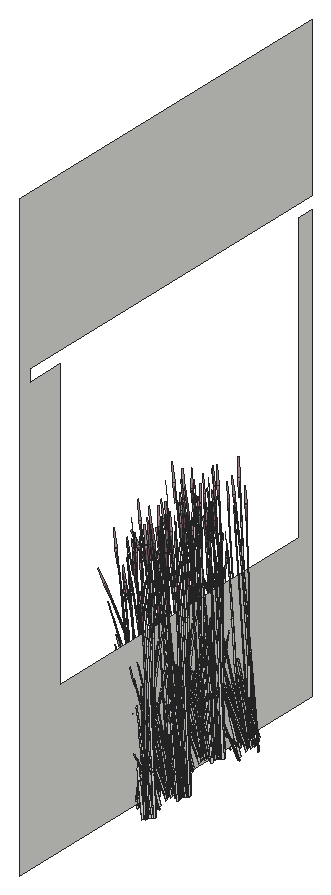
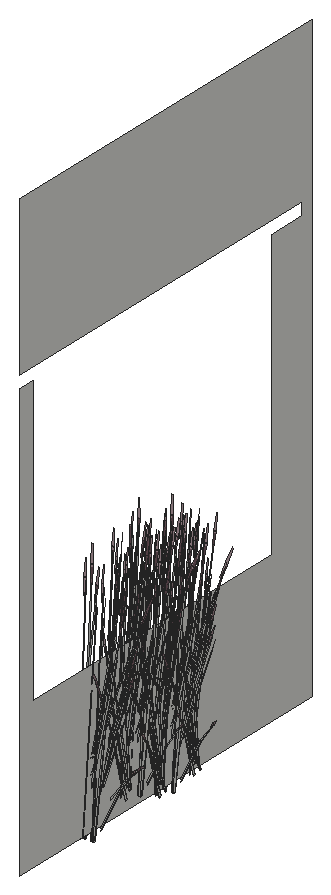
# SketchUp Ruby script. Lengths in inches.
U = 1.inch
M = Sketchup.active_model
def pt(a) = Geom::Point3d.new(a.map { |v| v * U })
def face(e, loops, mat)
  f = e.add_face(loops[0].map { |a| pt(a) })
  loops[1..].each { |l| e.add_face(l.map { |a| pt(a) }).erase! }
  f.material = f.back_material = mat if mat
  f
end
# faces: each face lists its corners as indices into pts; further lists are holes
def faces(e, pts, list, mat = nil) = list.each { |f| face(e, (f[0].is_a?(Array) ? f : [f]).map { |l| l.map { |i| pts[i] } }, mat) }
# xy, xz, yz: faces in a plane at the given z, y or x. An outline is a flat list of corners, or four numbers for a rectangle; further outlines are holes
def ring(l) = l.size == 4 ? [[l[0], l[1]], [l[2], l[1]], [l[2], l[3]], [l[0], l[3]]] : l.each_slice(2).to_a
def flat(e, list, mat, &to3) = list.each { |f| face(e, (f[0].is_a?(Array) ? f : [f]).map { |l| ring(l).map { |u, v| to3.(u, v) } }, mat) }
def xy(e, z, list, mat = nil) = flat(e, list, mat) { |x, y| [x, y, z] }
def xz(e, y, list, mat = nil) = flat(e, list, mat) { |x, z| [x, y, z] }
def yz(e, x, list, mat = nil) = flat(e, list, mat) { |y, z| [x, y, z] }
def lines(e, pts, list) = list.each { |a, b| e.add_line(pt(pts[a]), pt(pts[b])) }
# prism: a flat outline (further loops are holes) pulled along v
def prism(e, loops, v, mat = nil)
  f = face(e, loops, mat); d = Geom::Vector3d.new(v.map { |x| x * U })
  f.pushpull(f.normal.samedirection?(d) ? d.length : -d.length)
end
def box(e, o, s, mat = nil) = prism(e, [[o, [o[0] + s[0], o[1], o[2]], [o[0] + s[0], o[1] + s[1], o[2]], [o[0], o[1] + s[1], o[2]]]], [0, 0, s[2]], mat)
def at(x, y, z, deg = 0) = Geom::Transformation.translation(pt([x, y, z])) * Geom::Transformation.rotation(ORIGIN, Z_AXIS, deg.degrees)
def axes(o, x, y, z) = Geom::Transformation.new([*x, 0, *y, 0, *z, 0, *pt(o).to_a, 1])
def part(name) = M.definitions.add(name)
# library, detail: a bought-in or finely detailed component or shape, given as its bounding box
def library(name, o, s) = part(name).tap { |d| box(d.entities, o, s) }
def detail(e, o, s) = box(e.add_group.entities, o, s)
def put(e, d, t, mat = nil) = e.add_instance(d, t).tap { |i| i.material = mat if mat }
def group(e, t, mat = nil) = e.add_group.tap { |g| g.transformation = t; g.material = mat if mat }.entities
root = M.entities
M.materials.add("LightPink_Translucent").color = [144, 107, 117]
M.materials["LightPink_Translucent"].alpha = 0.75
c1 = part("blade")
p = [[2.15,0.21,22],[0,0.17,0],[0.09,0.45,0],[2.18,0.31,22],[2.29,0.31,22],[0.38,0.45,0],
  [2.48,0.24,33],[2.49,0.24,33],[2.48,0.22,33]]
faces(c1.entities,p,[[0,1,2,3],[4,5,2,3],[6,3,4,7],[8,0,3,6]])
c2 = part("seeds")
p = [[0.3,-0.1,1.38],[-0.01,-0.03,1.59],[-0.01,-0.03,0.03],[0.14,-0.07,-0.07],[0.29,-0.03,3],[0.15,0.01,3.11]]
faces(c2.entities,p,[[0,1,2,3],[1,0,4,5]],"LightPink_Translucent")
c3 = part("blade with seeds")
put(c3.entities,c1,at(0,0,0))
put(c3.entities,c2,axes([2.4,0.25,30.99],[1.5799,-0.05474,1.17369],[-0.12525,1.92788,0.29478],[-0.07173,-0.02425,1.56792]))
yz(root,342,[[51,6,138.72,6,138.72,111,135,111,135,42,63,42,63,111,54,111,54,114,138.72,114,138.72,151.99,51,151.99]])
put(root,c3,axes([345.8125,86.08,4.49],[-0.55235,-0.65609,-0.05142],[0.93577,-0.36461,0.51607],[-0.23059,0.06247,1.6363]))
put(root,c3,axes([345.62,84.5,4.91],[0.66093,0.39201,0.1448],[-0.5513,0.44227,-0.41347],[-0.15345,0.05979,1.26744]))
put(root,c3,axes([344.2,90.4,3.79],[-0.15005,0.02351,1.76342],[-0.82981,-0.26461,-0.26939],[0.01392,-0.22072,0.30037]))
put(root,c3,axes([346.32,85.7,4.77],[0.83726,-0.32623,0.49651],[0.50045,0.58498,0],[-0.19069,0.0743,1.57504]))
put(root,c3,axes([345.02,91.13,6.82],[0.2697,-0.50175,-0.35414],[0.78684,0.14635,0.4572],[-0.07215,-0.20201,0.87481]))
put(root,c3,axes([345.5625,86,4.32],[-0.83462,-0.16144,-0.30978],[0.21015,-0.56852,0.30978],[-0.16826,0.06556,1.38974]))
put(root,c3,axes([344.62,91.47,6.97],[-0.87941,-0.16356,-0.51099],[0.30143,-0.56078,-0.3958],[-0.08064,-0.22578,0.97773]))
put(root,c3,axes([345.42,84.35,4.96],[0.10425,0.7445,-0.29095],[-1.08575,0.04502,-0.50002],[-0.19119,0.09917,1.59708]))
put(root,c3,axes([342.87,91.12,7.39],[0.99656,-0.1677,0.53763],[0.17295,0.65785,0.4433],[-0.23438,-0.19388,1.11249]))
put(root,c3,axes([345.37,91.45,7.33],[-0.87543,0.30377,-0.1216],[-0.4302,-0.53915,-0.67495],[-0.1155,-0.2272,1.02557]))
put(root,c3,axes([341.89,90.53,5.06],[0.46666,0.22709,1.1486],[-0.67962,0.13651,0.84392],[-0.14541,-0.17452,0.25299]))
put(root,c3,axes([344.77,84.92,4.35],[-0.60257,0.49041,-0.62353],[-0.74854,-0.44469,-0.16365],[-0.24146,0.12234,1.37633]))
put(root,c3,axes([345.84,85.75,4.625],[1.11998,0.21207,0.30756],[-0.2802,0.75803,-0.36492],[-0.18537,0.09487,1.64885]))
put(root,c3,axes([345.76,86.26,4.3125],[-0.83726,0.32623,-0.49651],[-0.50045,-0.58498,0],[-0.19069,0.0743,1.57504]))
put(root,c3,axes([343.09,91.26,7.02],[0.4066,-0.41448,0.0643],[0.57901,0.24131,0.50621],[-0.18719,-0.13288,0.77189]))
put(root,c3,axes([342.97,93.57,4.39],[-0.36739,-0.66907,-0.69835],[1.05831,-0.24096,-0.18329],[-0.04061,-0.22656,1.54149]))
put(root,c3,axes([341.98,85.46,7.34],[0.60531,-0.34352,0.35414],[0.573,0.39225,-0.4572],[-0.08718,0.19929,0.87481]))
put(root,c3,axes([346.52,86.16,4.67],[0.55932,0.6538,0],[-0.93577,0.36461,-0.51607],[-0.21313,0.08304,1.63711]))
put(root,c3,axes([345.11,91.66,7.34],[-0.2697,0.50175,0.35414],[-0.78684,-0.14635,-0.4572],[-0.07215,-0.20201,0.87481]))
put(root,c3,axes([346.04,83.57,5.13],[-0.02444,-0.61432,1.41272],[1.10603,0.15924,0.59816],[-0.26159,0.33615,1.3335]))
put(root,c3,axes([344.05,90.86,4.42],[-0.61821,0.37431,-0.03893],[-0.56645,-0.40995,-0.17649],[-0.03988,-0.11616,0.58215]))
put(root,c3,axes([344.84,95.3,5.62],[0.77308,0.2631,1.51261],[-0.75736,0.56681,0.59816],[-0.33924,-0.33594,1.26806]))
put(root,c3,axes([343.22,91.74,7.34],[0.13817,0.52554,0.35414],[-0.78985,0.13877,-0.4572],[-0.21215,-0.1506,0.87481]))
put(root,c3,axes([340.8,93.48,4.3125],[0,-0.65246,-0.49651],[1.00089,0,0],[0,-0.1486,1.57504]))
put(root,c3,axes([343.4375,86.48,7.02],[-0.6592,0.22175,0.0643],[-0.32265,-0.40436,0.50621],[0.06366,0.17825,0.77189]))
put(root,c3,axes([341.67,85.95,6.82],[-0.60531,0.34352,-0.35414],[-0.573,-0.39225,0.4572],[-0.08718,0.19929,0.87481]))
put(root,c3,axes([341.6,85.56,7.69],[0.98321,0.03233,-0.13498],[-0.02687,0.61208,-0.74919],[-0.0683,0.23574,1.13838]))
put(root,c3,axes([343.67,86.4375,7.36],[-0.88151,-0.17057,0.53283],[0.30143,-0.56078,0.43934],[0.05297,0.22053,1.10256]))
put(root,c3,axes([342.05,87.28,5.06],[-0.02315,-0.38796,1.1486],[0.57853,0.27671,0.84392],[-0.11378,0.18492,0.25299]))
put(root,c3,axes([342.27,85.79,7.3],[0.64041,0.4384,-0.5672],[-0.67652,0.38394,-0.43934],[-0.09744,0.22274,1.08528]))
put(root,c3,axes([341.23,93.49,4.32],[0.62448,-0.40708,-0.30978],[0.62448,0.40708,0.30978],[0,-0.13112,1.38974]))
put(root,c3,axes([341.57,86.44,5.12],[0.8127,-0.11554,0.06507],[0.18684,0.46549,-0.86304],[-0.05152,0.23564,0.7736]))
put(root,c3,axes([343.42,94.23,4.96],[-1.00749,-0.31132,-0.29095],[0.48511,-0.65709,-0.50002],[-0.03166,-0.16133,1.59708]))
put(root,c3,axes([342.07,85.59,7.63],[-0.02328,0.60353,-0.7886],[-0.98022,-0.04053,0.09517],[-0.10344,0.25568,1.11556]))
put(root,c3,axes([339.51,87.17,7],[0.10149,-0.03939,1.77383],[0.83886,0.26202,-0.16761],[-0.01971,0.21816,0.31391]))
put(root,c3,axes([343,85.16,6.17],[-0.0219,-0.25042,1.71376],[0.94901,0.16613,0.13857],[-0.0587,0.35688,0.73262]))
put(root,c3,axes([341.42,93.78,4.625],[-0.83213,0.54855,0.30756],[-0.83263,-0.54278,-0.36492],[-0.02906,-0.15578,1.64885]))
put(root,c3,axes([343.67,94.92,4.73],[0.23711,-0.77313,-0.23429],[1.12425,0.13477,0.51271],[-0.19645,-0.10677,1.5644]))
put(root,c3,axes([341.23,94.08,4.77],[0,0.65246,0.49651],[-1.00089,0,0],[0,-0.1486,1.57504]))
put(root,c3,axes([341.74,86.44,5.66],[0.01966,-0.33682,1.54345],[0.88405,0.17791,0.21329],[-0.0766,0.35897,0.72882]))
put(root,c3,axes([343.59,94.61,4.5],[-0.53742,-0.54764,-0.44739],[0.81403,-0.38564,0.21531],[-0.17391,-0.06776,1.43643]))
put(root,c3,axes([343.7,93.84,4.65],[0.38895,0.72959,0.45755],[-1.11135,0.2537,0.17955],[0.01358,-0.13406,1.58856]))
put(root,c3,axes([343.51,94.41,5.01],[-0.43405,0.58792,0.44739],[-0.90188,-0.28295,-0.21531],[0,-0.13553,1.43643]))
put(root,c3,axes([345.38,94.48,4.59],[-0.83213,-0.56158,-0.06131],[0.83263,-0.56193,0],[-0.02906,-0.01961,1.75571]))
put(root,c3,axes([343.8,94.55,4.65],[1.13071,0.13747,0.45755],[-0.23011,0.77639,0.17955],[-0.16524,-0.07497,1.58856]))
put(root,c3,axes([343.19,95.79,4.77],[0.96132,-0.17317,0.17642],[0.23737,0.64447,0.35086],[-0.08574,-0.0939,1.60407]))
put(root,c3,axes([344.08,95.11,4.91],[-0.17258,0.58229,0.1448],[-0.84319,-0.10108,-0.41347],[-0.15345,-0.05979,1.26744]))
put(root,c3,axes([346.05,95.83,4.77],[0.25843,-0.64844,0.17642],[0.9457,0.1835,0.35086],[-0.16336,0.00316,1.60407]))
put(root,c3,axes([344.43,95.89,4.49],[-0.90188,-0.29293,0],[0.43405,-0.60866,0],[0,0,1.62707]))
put(root,c3,axes([345.18,95.12,4.76],[-0.87356,-0.52515,-0.25192],[0.73507,-0.5897,0.5513],[-0.23523,0.06143,1.68216]))
put(root,c3,axes([342.88,96.12,4.77],[0.83726,0.32623,0.49651],[-0.50045,0.58498,0],[-0.19069,-0.0743,1.57504]))
put(root,c3,axes([345.6,94.68,5.01],[0.97146,-0.04028,0.44739],[0.08785,0.66859,-0.21531],[-0.17391,0.06776,1.43643]))
put(root,c3,axes([344.74,95,4.5],[-0.97146,0.04028,-0.44739],[-0.08785,-0.66859,0.21531],[-0.17391,0.06776,1.43643]))
put(root,c3,axes([344.94,101.65,10.98],[-0.42698,-0.53052,-0.71045],[0.87893,-0.29566,0.08574],[-0.09984,-0.25633,1.00501]))
put(root,c3,axes([344.2,100.47,7.49],[-0.15005,0.02351,1.76342],[-0.82981,-0.26461,-0.26939],[0.01392,-0.22072,0.30037]))
put(root,c3,axes([345.8125,96.55,4.49],[-0.55235,-0.65609,-0.05142],[0.93577,-0.36461,0.51607],[-0.23059,0.06247,1.6363]))
put(root,c3,axes([345.62,94.97,4.91],[0.66093,0.39201,0.1448],[-0.5513,0.44227,-0.41347],[-0.15345,0.05979,1.26744]))
put(root,c3,axes([345.02,101.2,10.53],[0.2697,-0.50175,-0.35414],[0.78684,0.14635,0.4572],[-0.07215,-0.20201,0.87481]))
put(root,c3,axes([344.62,101.54,10.68],[-0.87941,-0.16356,-0.51099],[0.30143,-0.56078,-0.3958],[-0.08064,-0.22578,0.97773]))
put(root,c3,axes([346.32,96.18,4.77],[0.83726,-0.32623,0.49651],[0.50045,0.58498,0],[-0.19069,0.0743,1.57504]))
put(root,c3,axes([345.5625,96.47,4.32],[-0.83462,-0.16144,-0.30978],[0.21015,-0.56852,0.30978],[-0.16826,0.06556,1.38974]))
put(root,c3,axes([345.42,94.82,4.96],[0.10425,0.7445,-0.29095],[-1.08575,0.04502,-0.50002],[-0.19119,0.09917,1.59708]))
put(root,c3,axes([341.89,100.59,8.77],[0.46666,0.22709,1.1486],[-0.67962,0.13651,0.84392],[-0.14541,-0.17452,0.25299]))
put(root,c3,axes([344.77,95.39,4.35],[-0.60257,0.49041,-0.62353],[-0.74854,-0.44469,-0.16365],[-0.24146,0.12234,1.37633]))
put(root,c3,axes([345.84,96.22,4.625],[1.11998,0.21207,0.30756],[-0.2802,0.75803,-0.36492],[-0.18537,0.09487,1.64885]))
put(root,c3,axes([345.76,96.73,4.3125],[-0.83726,0.32623,-0.49651],[-0.50045,-0.58498,0],[-0.19069,0.0743,1.57504]))
put(root,c3,axes([342.97,103.64,8.1],[-0.36739,-0.66907,-0.69835],[1.05831,-0.24096,-0.18329],[-0.04061,-0.22656,1.54149]))
put(root,c3,axes([341.98,95.93,7.34],[0.60531,-0.34352,0.35414],[0.573,0.39225,-0.4572],[-0.08718,0.19929,0.87481]))
put(root,c3,axes([346.52,96.63,4.67],[0.55932,0.6538,0],[-0.93577,0.36461,-0.51607],[-0.21313,0.08304,1.63711]))
put(root,c3,axes([346.04,94.04,5.13],[-0.02444,-0.61432,1.41272],[1.10603,0.15924,0.59816],[-0.26159,0.33615,1.3335]))
put(root,c3,axes([344.05,100.93,8.13],[-0.61821,0.37431,-0.03893],[-0.56645,-0.40995,-0.17649],[-0.03988,-0.11616,0.58215]))
put(root,c3,axes([344.84,105.37,9.33],[0.77308,0.2631,1.51261],[-0.75736,0.56681,0.59816],[-0.33924,-0.33594,1.26806]))
put(root,c3,axes([340.8,103.55,8.02],[0,-0.65246,-0.49651],[1.00089,0,0],[0,-0.1486,1.57504]))
put(root,c3,axes([343.4375,96.95,7.02],[-0.6592,0.22175,0.0643],[-0.32265,-0.40436,0.50621],[0.06366,0.17825,0.77189]))
put(root,c3,axes([341.67,96.42,6.82],[-0.60531,0.34352,-0.35414],[-0.573,-0.39225,0.4572],[-0.08718,0.19929,0.87481]))
put(root,c3,axes([341.6,96.03,7.69],[0.98321,0.03233,-0.13498],[-0.02687,0.61208,-0.74919],[-0.0683,0.23574,1.13838]))
put(root,c3,axes([343.67,96.91,7.36],[-0.88151,-0.17057,0.53283],[0.30143,-0.56078,0.43934],[0.05297,0.22053,1.10256]))
put(root,c3,axes([342.05,97.75,5.06],[-0.02315,-0.38796,1.1486],[0.57853,0.27671,0.84392],[-0.11378,0.18492,0.25299]))
put(root,c3,axes([341.23,103.5625,8.03],[0.62448,-0.40708,-0.30978],[0.62448,0.40708,0.30978],[0,-0.13112,1.38974]))
put(root,c3,axes([343.42,104.3,8.67],[-1.00749,-0.31132,-0.29095],[0.48511,-0.65709,-0.50002],[-0.03166,-0.16133,1.59708]))
put(root,c3,axes([342.27,96.26,7.3],[0.64041,0.4384,-0.5672],[-0.67652,0.38394,-0.43934],[-0.09744,0.22274,1.08528]))
put(root,c3,axes([341.57,96.92,5.12],[0.8127,-0.11554,0.06507],[0.18684,0.46549,-0.86304],[-0.05152,0.23564,0.7736]))
put(root,c3,axes([342.07,96.06,7.63],[-0.02328,0.60353,-0.7886],[-0.98022,-0.04053,0.09517],[-0.10344,0.25568,1.11556]))
put(root,c3,axes([339.51,97.64,7],[0.10149,-0.03939,1.77383],[0.83886,0.26202,-0.16761],[-0.01971,0.21816,0.31391]))
put(root,c3,axes([341.42,103.85,8.33],[-0.83213,0.54855,0.30756],[-0.83263,-0.54278,-0.36492],[-0.02906,-0.15578,1.64885]))
put(root,c3,axes([343,95.63,6.17],[-0.0219,-0.25042,1.71376],[0.94901,0.16613,0.13857],[-0.0587,0.35688,0.73262]))
put(root,c3,axes([343.67,104.99,8.4375],[0.23711,-0.77313,-0.23429],[1.12425,0.13477,0.51271],[-0.19645,-0.10677,1.5644]))
put(root,c3,axes([341.23,104.15,8.48],[0,0.65246,0.49651],[-1.00089,0,0],[0,-0.1486,1.57504]))
put(root,c3,axes([343.59,104.68,8.21],[-0.53742,-0.54764,-0.44739],[0.81403,-0.38564,0.21531],[-0.17391,-0.06776,1.43643]))
put(root,c3,axes([343.7,103.91,8.36],[0.38895,0.72959,0.45755],[-1.11135,0.2537,0.17955],[0.01358,-0.13406,1.58856]))
put(root,c3,axes([343.51,104.48,8.72],[-0.43405,0.58792,0.44739],[-0.90188,-0.28295,-0.21531],[0,-0.13553,1.43643]))
put(root,c3,axes([341.74,96.91,5.66],[0.01966,-0.33682,1.54345],[0.88405,0.17791,0.21329],[-0.0766,0.35897,0.72882]))
put(root,c3,axes([345.38,104.55,8.3],[-0.83213,-0.56158,-0.06131],[0.83263,-0.56193,0],[-0.02906,-0.01961,1.75571]))
put(root,c3,axes([343.8,104.62,8.36],[1.13071,0.13747,0.45755],[-0.23011,0.77639,0.17955],[-0.16524,-0.07497,1.58856]))
put(root,c3,axes([343.19,105.86,8.47],[0.96132,-0.17317,0.17642],[0.23737,0.64447,0.35086],[-0.08574,-0.0939,1.60407]))
put(root,c3,axes([344.08,105.17,8.62],[-0.17258,0.58229,0.1448],[-0.84319,-0.10108,-0.41347],[-0.15345,-0.05979,1.26744]))
put(root,c3,axes([346.05,105.9,8.47],[0.25843,-0.64844,0.17642],[0.9457,0.1835,0.35086],[-0.16336,0.00316,1.60407]))
put(root,c3,axes([344.43,105.96,8.2],[-0.90188,-0.29293,0],[0.43405,-0.60866,0],[0,0,1.62707]))
put(root,c3,axes([345.18,105.18,8.46],[-0.87356,-0.52515,-0.25192],[0.73507,-0.5897,0.5513],[-0.23523,0.06143,1.68216]))
put(root,c3,axes([342.88,106.19,8.48],[0.83726,0.32623,0.49651],[-0.50045,0.58498,0],[-0.19069,-0.0743,1.57504]))
put(root,c3,axes([345.6,104.75,8.72],[0.97146,-0.04028,0.44739],[0.08785,0.66859,-0.21531],[-0.17391,0.06776,1.43643]))
put(root,c3,axes([344.74,105.07,8.21],[-0.97146,0.04028,-0.44739],[-0.08785,-0.66859,0.21531],[-0.17391,0.06776,1.43643]))
put(root,c3,axes([345.8125,106.62,8.19],[-0.55235,-0.65609,-0.05142],[0.93577,-0.36461,0.51607],[-0.23059,0.06247,1.6363]))
put(root,c3,axes([345.62,105.04,8.62],[0.66093,0.39201,0.1448],[-0.5513,0.44227,-0.41347],[-0.15345,0.05979,1.26744]))
put(root,c3,axes([346.32,106.24,8.48],[0.83726,-0.32623,0.49651],[0.50045,0.58498,0],[-0.19069,0.0743,1.57504]))
put(root,c3,axes([345.5625,106.54,8.03],[-0.83462,-0.16144,-0.30978],[0.21015,-0.56852,0.30978],[-0.16826,0.06556,1.38974]))
put(root,c3,axes([345.42,104.89,8.67],[0.10425,0.7445,-0.29095],[-1.08575,0.04502,-0.50002],[-0.19119,0.09917,1.59708]))
put(root,c3,axes([344.77,105.46,8.06],[-0.60257,0.49041,-0.62353],[-0.74854,-0.44469,-0.16365],[-0.24146,0.12234,1.37633]))
put(root,c3,axes([345.84,106.29,8.33],[1.11998,0.21207,0.30756],[-0.2802,0.75803,-0.36492],[-0.18537,0.09487,1.64885]))
put(root,c3,axes([345.76,106.8,8.02],[-0.83726,0.32623,-0.49651],[-0.50045,-0.58498,0],[-0.19069,0.0743,1.57504]))
put(root,c3,axes([346.52,106.7,8.375],[0.55932,0.6538,0],[-0.93577,0.36461,-0.51607],[-0.21313,0.08304,1.63711]))
put(root,c3,axes([346.04,104.11,8.84],[-0.02444,-0.61432,1.41272],[1.10603,0.15924,0.59816],[-0.26159,0.33615,1.3335]))
put(root,c3,axes([343.98,114.11,7.01],[-0.13683,-0.09148,1.74944],[-0.91315,0.058,-0.27667],[-0.14574,-0.2188,0.14031]))
put(root,c3,axes([344.94,115.65,7.27],[-0.42698,-0.53052,-0.71045],[0.87893,-0.29566,0.08574],[-0.09984,-0.25633,1.00501]))
put(root,c3,axes([344.2,114.48,3.79],[-0.15005,0.02351,1.76342],[-0.82981,-0.26461,-0.26939],[0.01392,-0.22072,0.30037]))
put(root,c3,axes([341.67,106.49,10.53],[-0.60531,0.34352,-0.35414],[-0.573,-0.39225,0.4572],[-0.08718,0.19929,0.87481]))
put(root,c3,axes([342.05,107.82,8.77],[-0.02315,-0.38796,1.1486],[0.57853,0.27671,0.84392],[-0.11378,0.18492,0.25299]))
put(root,c3,axes([345.02,115.2,6.82],[0.2697,-0.50175,-0.35414],[0.78684,0.14635,0.4572],[-0.07215,-0.20201,0.87481]))
put(root,c3,axes([342.27,106.32,11],[0.64041,0.4384,-0.5672],[-0.67652,0.38394,-0.43934],[-0.09744,0.22274,1.08528]))
put(root,c3,axes([344.62,115.55,6.97],[-0.87941,-0.16356,-0.51099],[0.30143,-0.56078,-0.3958],[-0.08064,-0.22578,0.97773]))
put(root,c3,axes([341.57,106.98,8.82],[0.8127,-0.11554,0.06507],[0.18684,0.46549,-0.86304],[-0.05152,0.23564,0.7736]))
put(root,c3,axes([342.87,115.2,7.39],[0.99656,-0.1677,0.53763],[0.17295,0.65785,0.4433],[-0.23438,-0.19388,1.11249]))
put(root,c3,axes([342.07,106.125,11.34],[-0.02328,0.60353,-0.7886],[-0.98022,-0.04053,0.09517],[-0.10344,0.25568,1.11556]))
put(root,c3,axes([345.37,115.52,7.33],[-0.87543,0.30377,-0.1216],[-0.4302,-0.53915,-0.67495],[-0.1155,-0.2272,1.02557]))
put(root,c3,axes([341.89,114.6,5.06],[0.46666,0.22709,1.1486],[-0.67962,0.13651,0.84392],[-0.14541,-0.17452,0.25299]))
put(root,c3,axes([343,105.7,9.875],[-0.0219,-0.25042,1.71376],[0.94901,0.16613,0.13857],[-0.0587,0.35688,0.73262]))
put(root,c3,axes([343.09,115.34,7.02],[0.4066,-0.41448,0.0643],[0.57901,0.24131,0.50621],[-0.18719,-0.13288,0.77189]))
put(root,c3,axes([342.97,117.65,4.39],[-0.36739,-0.66907,-0.69835],[1.05831,-0.24096,-0.18329],[-0.04061,-0.22656,1.54149]))
put(root,c3,axes([345.11,115.73,7.34],[-0.2697,0.50175,0.35414],[-0.78684,-0.14635,-0.4572],[-0.07215,-0.20201,0.87481]))
put(root,c3,axes([341.74,106.97,9.36],[0.01966,-0.33682,1.54345],[0.88405,0.17791,0.21329],[-0.0766,0.35897,0.72882]))
put(root,c3,axes([344.05,114.9375,4.42],[-0.61821,0.37431,-0.03893],[-0.56645,-0.40995,-0.17649],[-0.03988,-0.11616,0.58215]))
put(root,c3,axes([344.84,119.37,5.62],[0.77308,0.2631,1.51261],[-0.75736,0.56681,0.59816],[-0.33924,-0.33594,1.26806]))
put(root,c3,axes([343.22,115.82,7.34],[0.13817,0.52554,0.35414],[-0.78985,0.13877,-0.4572],[-0.21215,-0.1506,0.87481]))
put(root,c3,axes([340.8,117.55,4.3125],[0,-0.65246,-0.49651],[1.00089,0,0],[0,-0.1486,1.57504]))
put(root,c3,axes([341.23,117.57,4.32],[0.62448,-0.40708,-0.30978],[0.62448,0.40708,0.30978],[0,-0.13112,1.38974]))
put(root,c3,axes([343.42,118.31,4.96],[-1.00749,-0.31132,-0.29095],[0.48511,-0.65709,-0.50002],[-0.03166,-0.16133,1.59708]))
put(root,c3,axes([341.42,117.86,4.625],[-0.83213,0.54855,0.30756],[-0.83263,-0.54278,-0.36492],[-0.02906,-0.15578,1.64885]))
put(root,c3,axes([343.67,119,4.73],[0.23711,-0.77313,-0.23429],[1.12425,0.13477,0.51271],[-0.19645,-0.10677,1.5644]))
put(root,c3,axes([341.23,118.16,4.77],[0,0.65246,0.49651],[-1.00089,0,0],[0,-0.1486,1.57504]))
put(root,c3,axes([343.59,118.6875,4.5],[-0.53742,-0.54764,-0.44739],[0.81403,-0.38564,0.21531],[-0.17391,-0.06776,1.43643]))
put(root,c3,axes([343.7,117.91,4.65],[0.38895,0.72959,0.45755],[-1.11135,0.2537,0.17955],[0.01358,-0.13406,1.58856]))
put(root,c3,axes([343.51,118.49,5.01],[-0.43405,0.58792,0.44739],[-0.90188,-0.28295,-0.21531],[0,-0.13553,1.43643]))
put(root,c3,axes([345.38,118.56,4.59],[-0.83213,-0.56158,-0.06131],[0.83263,-0.56193,0],[-0.02906,-0.01961,1.75571]))
put(root,c3,axes([343.8,118.63,4.65],[1.13071,0.13747,0.45755],[-0.23011,0.77639,0.17955],[-0.16524,-0.07497,1.58856]))
